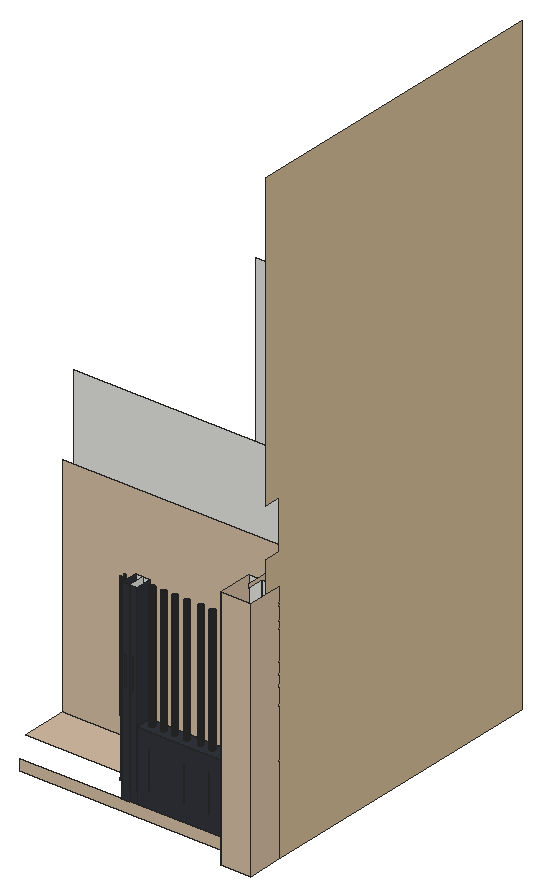
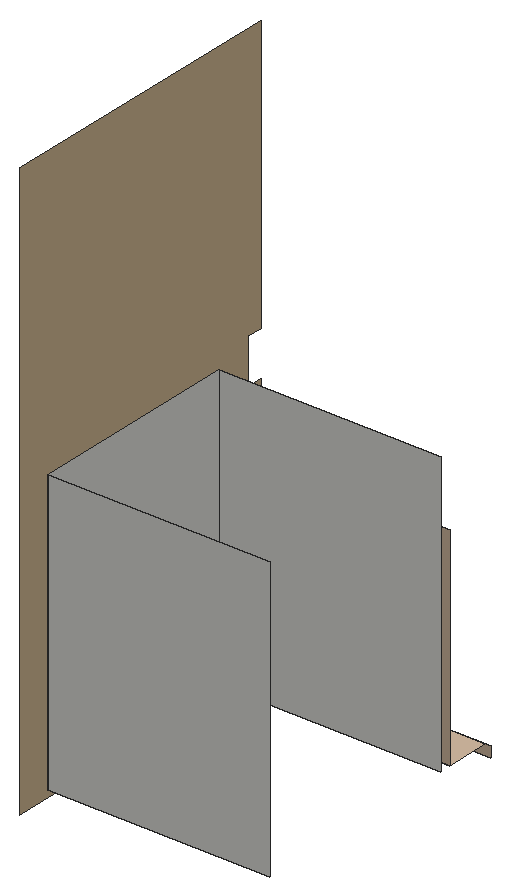
# SketchUp Ruby script. Lengths in inches.
U = 1.inch
M = Sketchup.active_model
def pt(a) = Geom::Point3d.new(a.map { |v| v * U })
def face(e, loops, mat)
  f = e.add_face(loops[0].map { |a| pt(a) })
  loops[1..].each { |l| e.add_face(l.map { |a| pt(a) }).erase! }
  f.material = f.back_material = mat if mat
  f
end
# faces: each face lists its corners as indices into pts; further lists are holes
def faces(e, pts, list, mat = nil) = list.each { |f| face(e, (f[0].is_a?(Array) ? f : [f]).map { |l| l.map { |i| pts[i] } }, mat) }
# xy, xz, yz: faces in a plane at the given z, y or x. An outline is a flat list of corners, or four numbers for a rectangle; further outlines are holes
def ring(l) = l.size == 4 ? [[l[0], l[1]], [l[2], l[1]], [l[2], l[3]], [l[0], l[3]]] : l.each_slice(2).to_a
def flat(e, list, mat, &to3) = list.each { |f| face(e, (f[0].is_a?(Array) ? f : [f]).map { |l| ring(l).map { |u, v| to3.(u, v) } }, mat) }
def xy(e, z, list, mat = nil) = flat(e, list, mat) { |x, y| [x, y, z] }
def xz(e, y, list, mat = nil) = flat(e, list, mat) { |x, z| [x, y, z] }
def yz(e, x, list, mat = nil) = flat(e, list, mat) { |y, z| [x, y, z] }
def lines(e, pts, list) = list.each { |a, b| e.add_line(pt(pts[a]), pt(pts[b])) }
# prism: a flat outline (further loops are holes) pulled along v
def prism(e, loops, v, mat = nil)
  f = face(e, loops, mat); d = Geom::Vector3d.new(v.map { |x| x * U })
  f.pushpull(f.normal.samedirection?(d) ? d.length : -d.length)
end
def box(e, o, s, mat = nil) = prism(e, [[o, [o[0] + s[0], o[1], o[2]], [o[0] + s[0], o[1] + s[1], o[2]], [o[0], o[1] + s[1], o[2]]]], [0, 0, s[2]], mat)
def at(x, y, z, deg = 0) = Geom::Transformation.translation(pt([x, y, z])) * Geom::Transformation.rotation(ORIGIN, Z_AXIS, deg.degrees)
def axes(o, x, y, z) = Geom::Transformation.new([*x, 0, *y, 0, *z, 0, *pt(o).to_a, 1])
def part(name) = M.definitions.add(name)
# library, detail: a bought-in or finely detailed component or shape, given as its bounding box
def library(name, o, s) = part(name).tap { |d| box(d.entities, o, s) }
def detail(e, o, s) = box(e.add_group.entities, o, s)
def put(e, d, t, mat = nil) = e.add_instance(d, t).tap { |i| i.material = mat if mat }
def group(e, t, mat = nil) = e.add_group.tap { |g| g.transformation = t; g.material = mat if mat }.entities
root = M.entities
M.materials.add("[Formica Beige]").color = [211, 187, 149]
M.materials.add("[Formica Laminate Dark]").color = [50, 53, 60]
M.materials.add("[Formica Laminate Light]").color = [213, 189, 164]
xy(root,9,[[213.5,71.93,213.24,71.96,213,72.0625,212.79,72.22,212.63,72.43,212.53,72.67,212.5,72.93,212.53,73.1875,212.63,73.43,212.79,73.63,213,73.79,213.24,73.89,213.5,73.93,213.76,73.89,214,73.79,214.21,73.63,214.37,73.43,214.46,73.1875,214.5,72.93,214.46,72.67,214.37,72.43,214.21,72.22,214,72.0625,213.76,71.96],[225.25,71.93,224.99,71.96,224.75,72.0625,224.54,72.22,224.38,72.43,224.28,72.67,224.25,72.93,224.28,73.1875,224.38,73.43,224.54,73.63,224.75,73.79,224.99,73.89,225.25,73.93,225.51,73.89,225.75,73.79,225.96,73.63,226.12,73.43,226.21,73.1875,226.25,72.93,226.21,72.67,226.12,72.43,225.96,72.22,225.75,72.0625,225.51,71.96],[229.8125,71.93,229.55,71.96,229.3125,72.0625,229.1,72.22,228.95,72.43,228.85,72.67,228.8125,72.93,228.85,73.1875,228.95,73.43,229.1,73.63,229.3125,73.79,229.55,73.89,229.8125,73.93,230.07,73.89,230.3125,73.79,230.52,73.63,230.68,73.43,230.78,73.1875,230.8125,72.93,230.78,72.67,230.68,72.43,230.52,72.22,230.3125,72.0625,230.07,71.96],[234.1875,71.93,233.93,71.96,233.6875,72.0625,233.48,72.22,233.32,72.43,233.22,72.67,233.1875,72.93,233.22,73.1875,233.32,73.43,233.48,73.63,233.6875,73.79,233.93,73.89,234.1875,73.93,234.45,73.89,234.6875,73.79,234.89,73.63,235.05,73.43,235.15,73.1875,235.1875,72.93,235.15,72.67,235.05,72.43,234.89,72.22,234.6875,72.0625,234.45,71.96],[239.1875,71.93,238.93,71.96,238.6875,72.0625,238.48,72.22,238.32,72.43,238.22,72.67,238.1875,72.93,238.22,73.1875,238.32,73.43,238.48,73.63,238.6875,73.79,238.93,73.89,239.1875,73.93,239.45,73.89,239.6875,73.79,239.89,73.63,240.05,73.43,240.15,73.1875,240.1875,72.93,240.15,72.67,240.05,72.43,239.89,72.22,239.6875,72.0625,239.45,71.96],
  [244.5625,71.93,244.3,71.96,244.0625,72.0625,243.85,72.22,243.7,72.43,243.6,72.67,243.5625,72.93,243.6,73.1875,243.7,73.43,243.85,73.63,244.0625,73.79,244.3,73.89,244.5625,73.93,244.82,73.89,245.0625,73.79,245.27,73.63,245.43,73.43,245.53,73.1875,245.5625,72.93,245.53,72.67,245.43,72.43,245.27,72.22,245.0625,72.0625,244.82,71.96],[249.3125,71.93,249.05,71.96,248.8125,72.0625,248.6,72.22,248.45,72.43,248.35,72.67,248.3125,72.93,248.35,73.1875,248.45,73.43,248.6,73.63,248.8125,73.79,249.05,73.89,249.3125,73.93,249.57,73.89,249.8125,73.79,250.02,73.63,250.18,73.43,250.28,73.1875,250.3125,72.93,250.28,72.67,250.18,72.43,250.02,72.22,249.8125,72.0625,249.57,71.96],[254.25,71.93,253.99,71.96,253.75,72.0625,253.54,72.22,253.38,72.43,253.28,72.67,253.25,72.93,253.28,73.1875,253.38,73.43,253.54,73.63,253.75,73.79,253.99,73.89,254.25,73.93,254.51,73.89,254.75,73.79,254.96,73.63,255.12,73.43,255.21,73.1875,255.25,72.93,255.21,72.67,255.12,72.43,254.96,72.22,254.75,72.0625,254.51,71.96],[258.6875,71.93,258.43,71.96,258.1875,72.0625,257.98,72.22,257.82,72.43,257.72,72.67,257.6875,72.93,257.72,73.1875,257.82,73.43,257.98,73.63,258.1875,73.79,258.43,73.89,258.6875,73.93,258.95,73.89,259.1875,73.79,259.39,73.63,259.55,73.43,259.65,73.1875,259.6875,72.93,259.65,72.67,259.55,72.43,259.39,72.22,259.1875,72.0625,258.95,71.96]])
xy(root,9,[[172.48,75.87,266.79,94.48]],"[Formica Laminate Light]")
xy(root,32.25,[[[221.95,69.35,261.51,75.87],[225.25,71.93,224.99,71.96,224.75,72.0625,224.54,72.22,224.38,72.43,224.28,72.67,224.25,72.93,224.28,73.1875,224.38,73.43,224.54,73.63,224.75,73.79,224.99,73.89,225.25,73.93,225.51,73.89,225.75,73.79,225.96,73.63,226.12,73.43,226.21,73.1875,226.25,72.93,226.21,72.67,226.12,72.43,225.96,72.22,225.75,72.0625,225.51,71.96],[229.8125,71.93,229.55,71.96,229.3125,72.0625,229.1,72.22,228.95,72.43,228.85,72.67,228.8125,72.93,228.85,73.1875,228.95,73.43,229.1,73.63,229.3125,73.79,229.55,73.89,229.8125,73.93,230.07,73.89,230.3125,73.79,230.52,73.63,230.68,73.43,230.78,73.1875,230.8125,72.93,230.78,72.67,230.68,72.43,230.52,72.22,230.3125,72.0625,230.07,71.96],[254.25,71.93,253.99,71.96,253.75,72.0625,253.54,72.22,253.38,72.43,253.28,72.67,253.25,72.93,253.28,73.1875,253.38,73.43,253.54,73.63,253.75,73.79,253.99,73.89,254.25,73.93,254.51,73.89,254.75,73.79,254.96,73.63,255.12,73.43,255.21,73.1875,255.25,72.93,255.21,72.67,255.12,72.43,254.96,72.22,254.75,72.0625,254.51,71.96],[234.1875,71.93,233.93,71.96,233.6875,72.0625,233.48,72.22,233.32,72.43,233.22,72.67,233.1875,72.93,233.22,73.1875,233.32,73.43,233.48,73.63,233.6875,73.79,233.93,73.89,234.1875,73.93,234.45,73.89,234.6875,73.79,234.89,73.63,235.05,73.43,235.15,73.1875,235.1875,72.93,235.15,72.67,235.05,72.43,234.89,72.22,234.6875,72.0625,234.45,71.96],[249.3125,71.93,249.05,71.96,248.8125,72.0625,248.6,72.22,248.45,72.43,248.35,72.67,248.3125,72.93,248.35,73.1875,248.45,73.43,248.6,73.63,248.8125,73.79,249.05,73.89,249.3125,73.93,249.57,73.89,249.8125,73.79,250.02,73.63,250.18,73.43,250.28,73.1875,250.3125,72.93,250.28,72.67,250.18,72.43,250.02,72.22,249.8125,72.0625,249.57,71.96],[239.1875,71.93,238.93,71.96,238.6875,72.0625,238.48,72.22,238.32,72.43,238.22,72.67,238.1875,72.93,238.22,73.1875,238.32,73.43,238.48,73.63,238.6875,73.79,238.93,73.89,239.1875,73.93,239.45,73.89,239.6875,73.79,239.89,73.63,240.05,73.43,240.15,73.1875,240.1875,72.93,240.15,72.67,240.05,72.43,239.89,72.22,239.6875,72.0625,239.45,71.96],[244.5625,71.93,244.3,71.96,244.0625,72.0625,243.85,72.22,243.7,72.43,243.6,72.67,243.5625,72.93,243.6,73.1875,243.7,73.43,243.85,73.63,244.0625,73.79,244.3,73.89,244.5625,73.93,244.82,73.89,245.0625,73.79,245.27,73.63,245.43,73.43,245.53,73.1875,245.5625,72.93,245.53,72.67,245.43,72.43,245.27,72.22,245.0625,72.0625,244.82,71.96],[258.6875,71.93,258.43,71.96,258.1875,72.0625,257.98,72.22,257.82,72.43,257.72,72.67,257.6875,72.93,257.72,73.1875,257.82,73.43,257.98,73.63,258.1875,73.79,258.43,73.89,258.6875,73.93,258.95,73.89,259.1875,73.79,259.39,73.63,259.55,73.43,259.65,73.1875,259.6875,72.93,259.65,72.67,259.55,72.43,259.39,72.22,259.1875,72.0625,258.95,71.96]]],"[Formica Laminate Dark]")
xz(root,61.98,[[261.51,0,273.31,97.5]],"[Formica Laminate Light]")
xz(root,69.35,[[[216.21,4.5,219.08,81.84],[216.72,44.27,217.85,56.83]],[[219.08,4.5,221.95,81.84],[219.85,44.27,220.97,56.83]],[221.95,4.5,261.51,32.25]],"[Formica Laminate Dark]")
xz(root,69.35,[[175.36,0,261.51,4.5]],"[Formica Laminate Light]")
xz(root,75.87,[[216.21,9,219.08,81.84],[219.08,9,221.95,81.84],[261.51,9,266.79,97.5],[266.79,9,273.31,97.5]])
xz(root,75.87,[[221.95,9,261.51,32.25]],"[Formica Laminate Dark]")
xz(root,94.48,[[172.48,9,266.79,98.95]],"[Formica Laminate Light]")
xz(root,99.67,[[172.48,9,266.79,129]])
xz(root,190.6,[[172.48,9,266.79,129]])
yz(root,216.21,[[69.35,9,75.87,32.25],[69.35,32.25,75.87,81.84]],"[Formica Laminate Dark]")
yz(root,219.08,[[69.35,9,75.87,81.84]])
yz(root,221.95,[[69.35,9,75.87,32.25],[69.35,32.25,75.87,81.84]],"[Formica Laminate Dark]")
yz(root,261.51,[[61.98,0,61.98,97.5,75.87,97.5,75.87,84.9,69.35,84.9,69.35,81.84,75.87,81.84,75.87,32.25,69.35,32.25,69.35,0]],"[Formica Laminate Light]")
yz(root,266.79,[[99.67,9,190.6,129]])
yz(root,266.79,[[75.87,9,75.87,97.5,69.35,97.5,69.35,98.95,94.48,98.95,94.48,9]],"[Formica Laminate Light]")
yz(root,273.31,[[75.87,0,197.12,0,197.12,246.5,69.35,246.5,69.35,129,75.87,129,75.87,109.89,69.35,109.89,69.35,97.5,75.87,97.5]],"[Formica Beige]")
yz(root,273.31,[[61.98,0,75.87,97.5]],"[Formica Laminate Light]")
p = [[213.5,71.93,9],[213.76,71.96,9],[213.76,71.96,32.25],[213.5,71.93,32.25],[224.99,71.96,9],[225.25,71.93,9],
  [225.25,71.93,32.25],[224.99,71.96,32.25],[225.51,71.96,9],[225.51,71.96,32.25],[229.55,71.96,9],[229.8125,71.93,9],
  [229.8125,71.93,32.25],[229.55,71.96,32.25],[230.07,71.96,9],[230.07,71.96,32.25],[233.93,71.96,9],[234.1875,71.93,9],
  [234.1875,71.93,32.25],[233.93,71.96,32.25],[234.45,71.96,9],[234.45,71.96,32.25],[238.93,71.96,9],[239.1875,71.93,9],
  [239.1875,71.93,32.25],[238.93,71.96,32.25],[239.45,71.96,9],[239.45,71.96,32.25],[244.3,71.96,9],[244.5625,71.93,9],
  [244.5625,71.93,32.25],[244.3,71.96,32.25],[244.82,71.96,9],[244.82,71.96,32.25],[249.05,71.96,9],[249.3125,71.93,9],
  [249.3125,71.93,32.25],[249.05,71.96,32.25],[249.57,71.96,9],[249.57,71.96,32.25],[253.99,71.96,9],[254.25,71.93,9],
  [254.25,71.93,32.25],[253.99,71.96,32.25],[254.51,71.96,9],[254.51,71.96,32.25],[258.43,71.96,9],[258.6875,71.93,9],
  [258.6875,71.93,32.25],[258.43,71.96,32.25],[258.95,71.96,9],[258.95,71.96,32.25],[214,72.0625,9],[214,72.0625,32.25],
  [224.75,72.0625,9],[224.75,72.0625,32.25],[225.75,72.0625,9],[225.75,72.0625,32.25],[229.3125,72.0625,9],[229.3125,72.0625,32.25],
  [230.3125,72.0625,9],[230.3125,72.0625,32.25],[233.6875,72.0625,9],[233.6875,72.0625,32.25],[234.6875,72.0625,9],[234.6875,72.0625,32.25],
  [238.6875,72.0625,9],[238.6875,72.0625,32.25],[239.6875,72.0625,9],[239.6875,72.0625,32.25],[244.0625,72.0625,9],[244.0625,72.0625,32.25],
  [245.0625,72.0625,9],[245.0625,72.0625,32.25],[248.8125,72.0625,9],[248.8125,72.0625,32.25],[249.8125,72.0625,9],[249.8125,72.0625,32.25],
  [253.75,72.0625,9],[253.75,72.0625,32.25],[254.75,72.0625,9],[254.75,72.0625,32.25],[258.1875,72.0625,9],[258.1875,72.0625,32.25],
  [259.1875,72.0625,9],[259.1875,72.0625,32.25],[214.21,72.22,9],[214.21,72.22,32.25],[224.54,72.22,9],[224.54,72.22,32.25],
  [225.96,72.22,9],[225.96,72.22,32.25],[229.1,72.22,9],[229.1,72.22,32.25],[230.52,72.22,9],[230.52,72.22,32.25],
  [233.48,72.22,9],[233.48,72.22,32.25],[234.89,72.22,9],[234.89,72.22,32.25],[238.48,72.22,9],[238.48,72.22,32.25],
  [239.89,72.22,9],[239.89,72.22,32.25],[243.85,72.22,9],[243.85,72.22,32.25],[245.27,72.22,9],[245.27,72.22,32.25],
  [248.6,72.22,9],[248.6,72.22,32.25],[250.02,72.22,9],[250.02,72.22,32.25],[253.54,72.22,9],[253.54,72.22,32.25],
  [254.96,72.22,9],[254.96,72.22,32.25],[257.98,72.22,9],[257.98,72.22,32.25],[259.39,72.22,9],[259.39,72.22,32.25],
  [214.37,72.43,9],[214.37,72.43,32.25],[224.38,72.43,9],[224.38,72.43,32.25],[226.12,72.43,9],[226.12,72.43,32.25],
  [228.95,72.43,9],[228.95,72.43,32.25],[230.68,72.43,9],[230.68,72.43,32.25],[233.32,72.43,9],[233.32,72.43,32.25],
  [235.05,72.43,9],[235.05,72.43,32.25],[238.32,72.43,9],[238.32,72.43,32.25],[240.05,72.43,9],[240.05,72.43,32.25],
  [243.7,72.43,9],[243.7,72.43,32.25],[245.43,72.43,9],[245.43,72.43,32.25],[248.45,72.43,9],[248.45,72.43,32.25],
  [250.18,72.43,9],[250.18,72.43,32.25],[253.38,72.43,9],[253.38,72.43,32.25],[255.12,72.43,9],[255.12,72.43,32.25],
  [257.82,72.43,9],[257.82,72.43,32.25],[259.55,72.43,9],[259.55,72.43,32.25],[214.46,72.67,9],[214.46,72.67,32.25],
  [224.28,72.67,9],[224.28,72.67,32.25],[226.21,72.67,9],[226.21,72.67,32.25],[228.85,72.67,9],[228.85,72.67,32.25],
  [230.78,72.67,9],[230.78,72.67,32.25],[233.22,72.67,9],[233.22,72.67,32.25],[235.15,72.67,9],[235.15,72.67,32.25],
  [238.22,72.67,9],[238.22,72.67,32.25],[240.15,72.67,9],[240.15,72.67,32.25],[243.6,72.67,9],[243.6,72.67,32.25],
  [245.53,72.67,9],[245.53,72.67,32.25],[248.35,72.67,9],[248.35,72.67,32.25],[250.28,72.67,9],[250.28,72.67,32.25],
  [253.28,72.67,9],[253.28,72.67,32.25],[255.21,72.67,9],[255.21,72.67,32.25],[257.72,72.67,9],[257.72,72.67,32.25],
  [259.65,72.67,9],[259.65,72.67,32.25],[214.5,72.93,9],[214.5,72.93,32.25],[224.25,72.93,9],[224.25,72.93,32.25],
  [226.25,72.93,9],[226.25,72.93,32.25],[228.8125,72.93,9],[228.8125,72.93,32.25],[230.8125,72.93,9],[230.8125,72.93,32.25],
  [233.1875,72.93,9],[233.1875,72.93,32.25],[235.1875,72.93,9],[235.1875,72.93,32.25],[238.1875,72.93,9],[238.1875,72.93,32.25],
  [240.1875,72.93,9],[240.1875,72.93,32.25],[243.5625,72.93,9],[243.5625,72.93,32.25],[245.5625,72.93,9],[245.5625,72.93,32.25],
  [248.3125,72.93,9],[248.3125,72.93,32.25],[250.3125,72.93,9],[250.3125,72.93,32.25],[253.25,72.93,9],[253.25,72.93,32.25],
  [255.25,72.93,9],[255.25,72.93,32.25],[257.6875,72.93,9],[257.6875,72.93,32.25],[259.6875,72.93,9],[259.6875,72.93,32.25],
  [214.46,73.1875,9],[214.46,73.1875,32.25],[224.28,73.1875,9],[224.28,73.1875,32.25],[226.21,73.1875,9],[226.21,73.1875,32.25],
  [228.85,73.1875,9],[228.85,73.1875,32.25],[230.78,73.1875,9],[230.78,73.1875,32.25],[233.22,73.1875,9],[233.22,73.1875,32.25],
  [235.15,73.1875,9],[235.15,73.1875,32.25],[238.22,73.1875,9],[238.22,73.1875,32.25],[240.15,73.1875,9],[240.15,73.1875,32.25],
  [243.6,73.1875,9],[243.6,73.1875,32.25],[245.53,73.1875,9],[245.53,73.1875,32.25],[248.35,73.1875,9],[248.35,73.1875,32.25],
  [250.28,73.1875,9],[250.28,73.1875,32.25],[253.28,73.1875,9],[253.28,73.1875,32.25],[255.21,73.1875,9],[255.21,73.1875,32.25],
  [257.72,73.1875,9],[257.72,73.1875,32.25],[259.65,73.1875,9],[259.65,73.1875,32.25],[214.37,73.43,9],[214.37,73.43,32.25],
  [224.38,73.43,9],[224.38,73.43,32.25],[226.12,73.43,9],[226.12,73.43,32.25],[228.95,73.43,9],[228.95,73.43,32.25],
  [230.68,73.43,9],[230.68,73.43,32.25],[233.32,73.43,9],[233.32,73.43,32.25],[235.05,73.43,9],[235.05,73.43,32.25],
  [238.32,73.43,9],[238.32,73.43,32.25],[240.05,73.43,9],[240.05,73.43,32.25],[243.7,73.43,9],[243.7,73.43,32.25],
  [245.43,73.43,9],[245.43,73.43,32.25],[248.45,73.43,9],[248.45,73.43,32.25],[250.18,73.43,9],[250.18,73.43,32.25],
  [253.38,73.43,9],[253.38,73.43,32.25],[255.12,73.43,9],[255.12,73.43,32.25],[257.82,73.43,9],[257.82,73.43,32.25],
  [259.55,73.43,9],[259.55,73.43,32.25],[214.21,73.63,9],[214.21,73.63,32.25],[224.54,73.63,9],[224.54,73.63,32.25],
  [225.96,73.63,9],[225.96,73.63,32.25],[229.1,73.63,9],[229.1,73.63,32.25],[230.52,73.63,9],[230.52,73.63,32.25],
  [233.48,73.63,9],[233.48,73.63,32.25],[234.89,73.63,9],[234.89,73.63,32.25],[238.48,73.63,9],[238.48,73.63,32.25],
  [239.89,73.63,9],[239.89,73.63,32.25],[243.85,73.63,9],[243.85,73.63,32.25],[245.27,73.63,9],[245.27,73.63,32.25],
  [248.6,73.63,9],[248.6,73.63,32.25],[250.02,73.63,9],[250.02,73.63,32.25],[253.54,73.63,9],[253.54,73.63,32.25],
  [254.96,73.63,9],[254.96,73.63,32.25],[257.98,73.63,9],[257.98,73.63,32.25],[259.39,73.63,9],[259.39,73.63,32.25],
  [214,73.79,9],[214,73.79,32.25],[224.75,73.79,9],[224.75,73.79,32.25],[225.75,73.79,9],[225.75,73.79,32.25],
  [229.3125,73.79,9],[229.3125,73.79,32.25],[230.3125,73.79,9],[230.3125,73.79,32.25],[233.6875,73.79,9],[233.6875,73.79,32.25],
  [234.6875,73.79,9],[234.6875,73.79,32.25],[238.6875,73.79,9],[238.6875,73.79,32.25],[239.6875,73.79,9],[239.6875,73.79,32.25],
  [244.0625,73.79,9],[244.0625,73.79,32.25],[245.0625,73.79,9],[245.0625,73.79,32.25],[248.8125,73.79,9],[248.8125,73.79,32.25],
  [249.8125,73.79,9],[249.8125,73.79,32.25],[253.75,73.79,9],[253.75,73.79,32.25],[254.75,73.79,9],[254.75,73.79,32.25],
  [258.1875,73.79,9],[258.1875,73.79,32.25],[259.1875,73.79,9],[259.1875,73.79,32.25],[213.76,73.89,9],[213.76,73.89,32.25],
  [224.99,73.89,9],[224.99,73.89,32.25],[225.51,73.89,9],[225.51,73.89,32.25],[229.55,73.89,9],[229.55,73.89,32.25],
  [230.07,73.89,9],[230.07,73.89,32.25],[233.93,73.89,9],[233.93,73.89,32.25],[234.45,73.89,9],[234.45,73.89,32.25],
  [238.93,73.89,9],[238.93,73.89,32.25],[239.45,73.89,9],[239.45,73.89,32.25],[244.3,73.89,9],[244.3,73.89,32.25],
  [244.82,73.89,9],[244.82,73.89,32.25],[249.05,73.89,9],[249.05,73.89,32.25],[249.57,73.89,9],[249.57,73.89,32.25],
  [253.99,73.89,9],[253.99,73.89,32.25],[254.51,73.89,9],[254.51,73.89,32.25],[258.43,73.89,9],[258.43,73.89,32.25],
  [258.95,73.89,9],[258.95,73.89,32.25],[213.5,73.93,9],[213.5,73.93,32.25],[225.25,73.93,9],[225.25,73.93,32.25],
  [229.8125,73.93,9],[229.8125,73.93,32.25],[234.1875,73.93,9],[234.1875,73.93,32.25],[239.1875,73.93,9],[239.1875,73.93,32.25],
  [244.5625,73.93,9],[244.5625,73.93,32.25],[249.3125,73.93,9],[249.3125,73.93,32.25],[254.25,73.93,9],[254.25,73.93,32.25],
  [258.6875,73.93,9],[258.6875,73.93,32.25],[213.24,71.96,81.84],[213.24,71.96,32.25],[213.5,71.93,81.84],[213.76,71.96,81.84],
  [224.99,71.96,81.84],[225.25,71.93,81.84],[225.51,71.96,81.84],[229.55,71.96,81.84],[229.8125,71.93,81.84],[230.07,71.96,81.84],
  [233.93,71.96,81.84],[234.1875,71.93,81.84],[234.45,71.96,81.84],[238.93,71.96,81.84],[239.1875,71.93,81.84],[239.45,71.96,81.84],
  [244.3,71.96,81.84],[244.5625,71.93,81.84],[244.82,71.96,81.84],[249.05,71.96,81.84],[249.3125,71.93,81.84],[249.57,71.96,81.84],
  [253.99,71.96,81.84],[254.25,71.93,81.84],[254.51,71.96,81.84],[258.43,71.96,81.84],[258.6875,71.93,81.84],[258.95,71.96,81.84],
  [214,72.0625,81.84],[224.75,72.0625,81.84],[225.75,72.0625,81.84],[229.3125,72.0625,81.84],[230.3125,72.0625,81.84],[233.6875,72.0625,81.84],
  [234.6875,72.0625,81.84],[238.6875,72.0625,81.84],[239.6875,72.0625,81.84],[244.0625,72.0625,81.84],[245.0625,72.0625,81.84],[248.8125,72.0625,81.84],
  [249.8125,72.0625,81.84],[253.75,72.0625,81.84],[254.75,72.0625,81.84],[258.1875,72.0625,81.84],[259.1875,72.0625,81.84],[214.21,72.22,81.84],
  [224.54,72.22,81.84],[225.96,72.22,81.84],[229.1,72.22,81.84],[230.52,72.22,81.84],[233.48,72.22,81.84],[234.89,72.22,81.84],
  [238.48,72.22,81.84],[239.89,72.22,81.84],[243.85,72.22,81.84],[245.27,72.22,81.84],[248.6,72.22,81.84],[250.02,72.22,81.84],
  [253.54,72.22,81.84],[254.96,72.22,81.84],[257.98,72.22,81.84],[259.39,72.22,81.84],[214.37,72.43,81.84],[224.38,72.43,81.84],
  [226.12,72.43,81.84],[228.95,72.43,81.84],[230.68,72.43,81.84],[233.32,72.43,81.84],[235.05,72.43,81.84],[238.32,72.43,81.84],
  [240.05,72.43,81.84],[243.7,72.43,81.84],[245.43,72.43,81.84],[248.45,72.43,81.84],[250.18,72.43,81.84],[253.38,72.43,81.84],
  [255.12,72.43,81.84],[257.82,72.43,81.84],[259.55,72.43,81.84],[214.46,72.67,81.84],[224.28,72.67,81.84],[226.21,72.67,81.84],
  [228.85,72.67,81.84],[230.78,72.67,81.84],[233.22,72.67,81.84],[235.15,72.67,81.84],[238.22,72.67,81.84],[240.15,72.67,81.84],
  [243.6,72.67,81.84],[245.53,72.67,81.84],[248.35,72.67,81.84],[250.28,72.67,81.84],[253.28,72.67,81.84],[255.21,72.67,81.84],
  [257.72,72.67,81.84],[259.65,72.67,81.84],[214.5,72.93,81.84],[224.25,72.93,81.84],[226.25,72.93,81.84],[228.8125,72.93,81.84],
  [230.8125,72.93,81.84],[233.1875,72.93,81.84],[235.1875,72.93,81.84],[238.1875,72.93,81.84],[240.1875,72.93,81.84],[243.5625,72.93,81.84],
  [245.5625,72.93,81.84],[248.3125,72.93,81.84],[250.3125,72.93,81.84],[253.25,72.93,81.84],[255.25,72.93,81.84],[257.6875,72.93,81.84],
  [259.6875,72.93,81.84],[214.46,73.1875,81.84],[224.28,73.1875,81.84],[226.21,73.1875,81.84],[228.85,73.1875,81.84],[230.78,73.1875,81.84],
  [233.22,73.1875,81.84],[235.15,73.1875,81.84],[238.22,73.1875,81.84],[240.15,73.1875,81.84],[243.6,73.1875,81.84],[245.53,73.1875,81.84],
  [248.35,73.1875,81.84],[250.28,73.1875,81.84],[253.28,73.1875,81.84],[255.21,73.1875,81.84],[257.72,73.1875,81.84],[259.65,73.1875,81.84],
  [214.37,73.43,81.84],[224.38,73.43,81.84],[226.12,73.43,81.84],[228.95,73.43,81.84],[230.68,73.43,81.84],[233.32,73.43,81.84],
  [235.05,73.43,81.84],[238.32,73.43,81.84],[240.05,73.43,81.84],[243.7,73.43,81.84],[245.43,73.43,81.84],[248.45,73.43,81.84],
  [250.18,73.43,81.84],[253.38,73.43,81.84],[255.12,73.43,81.84],[257.82,73.43,81.84],[259.55,73.43,81.84],[214.21,73.63,81.84],
  [224.54,73.63,81.84],[225.96,73.63,81.84],[229.1,73.63,81.84],[230.52,73.63,81.84],[233.48,73.63,81.84],[234.89,73.63,81.84],
  [238.48,73.63,81.84],[239.89,73.63,81.84],[243.85,73.63,81.84],[245.27,73.63,81.84],[248.6,73.63,81.84],[250.02,73.63,81.84],
  [253.54,73.63,81.84],[254.96,73.63,81.84],[257.98,73.63,81.84],[259.39,73.63,81.84],[214,73.79,81.84],[224.75,73.79,81.84],
  [225.75,73.79,81.84],[229.3125,73.79,81.84],[230.3125,73.79,81.84],[233.6875,73.79,81.84],[234.6875,73.79,81.84],[238.6875,73.79,81.84],
  [239.6875,73.79,81.84],[244.0625,73.79,81.84],[245.0625,73.79,81.84],[248.8125,73.79,81.84],[249.8125,73.79,81.84],[253.75,73.79,81.84],
  [254.75,73.79,81.84],[258.1875,73.79,81.84],[259.1875,73.79,81.84],[213.76,73.89,81.84],[224.99,73.89,81.84],[225.51,73.89,81.84],
  [229.55,73.89,81.84],[230.07,73.89,81.84],[233.93,73.89,81.84],[234.45,73.89,81.84],[238.93,73.89,81.84],[239.45,73.89,81.84],
  [244.3,73.89,81.84],[244.82,73.89,81.84],[249.05,73.89,81.84],[249.57,73.89,81.84],[253.99,73.89,81.84],[254.51,73.89,81.84],
  [258.43,73.89,81.84],[258.95,73.89,81.84],[213.5,73.93,81.84],[213.24,73.89,32.25],[213.24,73.89,81.84],[225.25,73.93,81.84],
  [229.8125,73.93,81.84],[234.1875,73.93,81.84],[239.1875,73.93,81.84],[244.5625,73.93,81.84],[249.3125,73.93,81.84],[254.25,73.93,81.84],
  [258.6875,73.93,81.84]]
faces(root,p,[[0,1,2,3],[4,5,6,7],[5,8,9,6],[10,11,12,13],[11,14,15,12],[16,17,18,19],[17,20,21,18],[22,23,24,25],
  [23,26,27,24],[28,29,30,31],[29,32,33,30],[34,35,36,37],[35,38,39,36],[40,41,42,43],[41,44,45,42],[46,47,48,49],
  [47,50,51,48],[1,52,53,2],[54,4,7,55],[8,56,57,9],[58,10,13,59],[14,60,61,15],[62,16,19,63],[20,64,65,21],
  [66,22,25,67],[26,68,69,27],[70,28,31,71],[32,72,73,33],[74,34,37,75],[38,76,77,39],[78,40,43,79],[44,80,81,45],
  [82,46,49,83],[50,84,85,51],[52,86,87,53],[88,54,55,89],[56,90,91,57],[92,58,59,93],[60,94,95,61],[96,62,63,97],
  [64,98,99,65],[100,66,67,101],[68,102,103,69],[104,70,71,105],[72,106,107,73],[108,74,75,109],[76,110,111,77],[112,78,79,113],
  [80,114,115,81],[116,82,83,117],[84,118,119,85],[86,120,121,87],[122,88,89,123],[90,124,125,91],[126,92,93,127],[94,128,129,95],
  [130,96,97,131],[98,132,133,99],[134,100,101,135],[102,136,137,103],[138,104,105,139],[106,140,141,107],[142,108,109,143],[110,144,145,111],
  [146,112,113,147],[114,148,149,115],[150,116,117,151],[118,152,153,119],[120,154,155,121],[156,122,123,157],[124,158,159,125],[160,126,127,161],
  [128,162,163,129],[164,130,131,165],[132,166,167,133],[168,134,135,169],[136,170,171,137],[172,138,139,173],[140,174,175,141],[176,142,143,177],
  [144,178,179,145],[180,146,147,181],[148,182,183,149],[184,150,151,185],[152,186,187,153],[154,188,189,155],[190,156,157,191],[158,192,193,159],
  [194,160,161,195],[162,196,197,163],[198,164,165,199],[166,200,201,167],[202,168,169,203],[170,204,205,171],[206,172,173,207],[174,208,209,175],
  [210,176,177,211],[178,212,213,179],[214,180,181,215],[182,216,217,183],[218,184,185,219],[186,220,221,187],[188,222,223,189],[224,190,191,225],
  [192,226,227,193],[228,194,195,229],[196,230,231,197],[232,198,199,233],[200,234,235,201],[236,202,203,237],[204,238,239,205],[240,206,207,241],
  [208,242,243,209],[244,210,211,245],[212,246,247,213],[248,214,215,249],[216,250,251,217],[252,218,219,253],[220,254,255,221],[222,256,257,223],
  [258,224,225,259],[226,260,261,227],[262,228,229,263],[230,264,265,231],[266,232,233,267],[234,268,269,235],[270,236,237,271],[238,272,273,239],
  [274,240,241,275],[242,276,277,243],[278,244,245,279],[246,280,281,247],[282,248,249,283],[250,284,285,251],[286,252,253,287],[254,288,289,255],
  [256,290,291,257],[292,258,259,293],[260,294,295,261],[296,262,263,297],[264,298,299,265],[300,266,267,301],[268,302,303,269],[304,270,271,305],
  [272,306,307,273],[308,274,275,309],[276,310,311,277],[312,278,279,313],[280,314,315,281],[316,282,283,317],[284,318,319,285],[320,286,287,321],
  [288,322,323,289],[290,324,325,291],[326,292,293,327],[294,328,329,295],[330,296,297,331],[298,332,333,299],[334,300,301,335],[302,336,337,303],
  [338,304,305,339],[306,340,341,307],[342,308,309,343],[310,344,345,311],[346,312,313,347],[314,348,349,315],[350,316,317,351],[318,352,353,319],
  [354,320,321,355],[322,356,357,323],[324,358,359,325],[360,326,327,361],[328,362,363,329],[364,330,331,365],[332,366,367,333],[368,334,335,369],
  [336,370,371,337],[372,338,339,373],[340,374,375,341],[376,342,343,377],[344,378,379,345],[380,346,347,381],[348,382,383,349],[384,350,351,385],
  [352,386,387,353],[388,354,355,389],[356,390,391,357],[358,392,393,359],[394,360,361,395],[362,394,395,363],[396,364,365,397],[366,396,397,367],
  [398,368,369,399],[370,398,399,371],[400,372,373,401],[374,400,401,375],[402,376,377,403],[378,402,403,379],[404,380,381,405],[382,404,405,383],
  [406,384,385,407],[386,406,407,387],[408,388,389,409],[390,408,409,391],[410,411,3,412],[412,3,2,413],[414,7,6,415],[415,6,9,416],
  [417,13,12,418],[418,12,15,419],[420,19,18,421],[421,18,21,422],[423,25,24,424],[424,24,27,425],[426,31,30,427],[427,30,33,428],
  [429,37,36,430],[430,36,39,431],[432,43,42,433],[433,42,45,434],[435,49,48,436],[436,48,51,437],[413,2,53,438],[439,55,7,414],
  [416,9,57,440],[441,59,13,417],[419,15,61,442],[443,63,19,420],[422,21,65,444],[445,67,25,423],[425,27,69,446],[447,71,31,426],
  [428,33,73,448],[449,75,37,429],[431,39,77,450],[451,79,43,432],[434,45,81,452],[453,83,49,435],[437,51,85,454],[438,53,87,455],
  [456,89,55,439],[440,57,91,457],[458,93,59,441],[442,61,95,459],[460,97,63,443],[444,65,99,461],[462,101,67,445],[446,69,103,463],
  [464,105,71,447],[448,73,107,465],[466,109,75,449],[450,77,111,467],[468,113,79,451],[452,81,115,469],[470,117,83,453],[454,85,119,471],
  [455,87,121,472],[473,123,89,456],[457,91,125,474],[475,127,93,458],[459,95,129,476],[477,131,97,460],[461,99,133,478],[479,135,101,462],
  [463,103,137,480],[481,139,105,464],[465,107,141,482],[483,143,109,466],[467,111,145,484],[485,147,113,468],[469,115,149,486],[487,151,117,470],
  [471,119,153,488],[472,121,155,489],[490,157,123,473],[474,125,159,491],[492,161,127,475],[476,129,163,493],[494,165,131,477],[478,133,167,495],
  [496,169,135,479],[480,137,171,497],[498,173,139,481],[482,141,175,499],[500,177,143,483],[484,145,179,501],[502,181,147,485],[486,149,183,503],
  [504,185,151,487],[488,153,187,505],[489,155,189,506],[507,191,157,490],[491,159,193,508],[509,195,161,492],[493,163,197,510],[511,199,165,494],
  [495,167,201,512],[513,203,169,496],[497,171,205,514],[515,207,173,498],[499,175,209,516],[517,211,177,500],[501,179,213,518],[519,215,181,502],
  [503,183,217,520],[521,219,185,504],[505,187,221,522],[506,189,223,523],[524,225,191,507],[508,193,227,525],[526,229,195,509],[510,197,231,527],
  [528,233,199,511],[512,201,235,529],[530,237,203,513],[514,205,239,531],[532,241,207,515],[516,209,243,533],[534,245,211,517],[518,213,247,535],
  [536,249,215,519],[520,217,251,537],[538,253,219,521],[522,221,255,539],[523,223,257,540],[541,259,225,524],[525,227,261,542],[543,263,229,526],
  [527,231,265,544],[545,267,233,528],[529,235,269,546],[547,271,237,530],[531,239,273,548],[549,275,241,532],[533,243,277,550],[551,279,245,534],
  [535,247,281,552],[553,283,249,536],[537,251,285,554],[555,287,253,538],[539,255,289,556],[540,257,291,557],[558,293,259,541],[542,261,295,559],
  [560,297,263,543],[544,265,299,561],[562,301,267,545],[546,269,303,563],[564,305,271,547],[548,273,307,565],[566,309,275,549],[550,277,311,567],
  [568,313,279,551],[552,281,315,569],[570,317,283,553],[554,285,319,571],[572,321,287,555],[556,289,323,573],[557,291,325,574],[575,327,293,558],
  [559,295,329,576],[577,331,297,560],[561,299,333,578],[579,335,301,562],[563,303,337,580],[581,339,305,564],[565,307,341,582],[583,343,309,566],
  [567,311,345,584],[585,347,313,568],[569,315,349,586],[587,351,317,570],[571,319,353,588],[589,355,321,572],[573,323,357,590],[574,325,359,591],
  [592,361,327,575],[576,329,363,593],[594,365,331,577],[578,333,367,595],[596,369,335,579],[580,337,371,597],[598,373,339,581],[582,341,375,599],
  [600,377,343,583],[584,345,379,601],[602,381,347,585],[586,349,383,603],[604,385,351,587],[588,353,387,605],[606,389,355,589],[590,357,391,607],
  [608,393,609,610],[591,359,393,608],[611,395,361,592],[593,363,395,611],[612,397,365,594],[595,367,397,612],[613,399,369,596],[597,371,399,613],
  [614,401,373,598],[599,375,401,614],[615,403,377,600],[601,379,403,615],[616,405,381,602],[603,383,405,616],[617,407,385,604],[605,387,407,617],
  [618,409,389,606],[607,391,409,618]],"[Formica Laminate Dark]")
